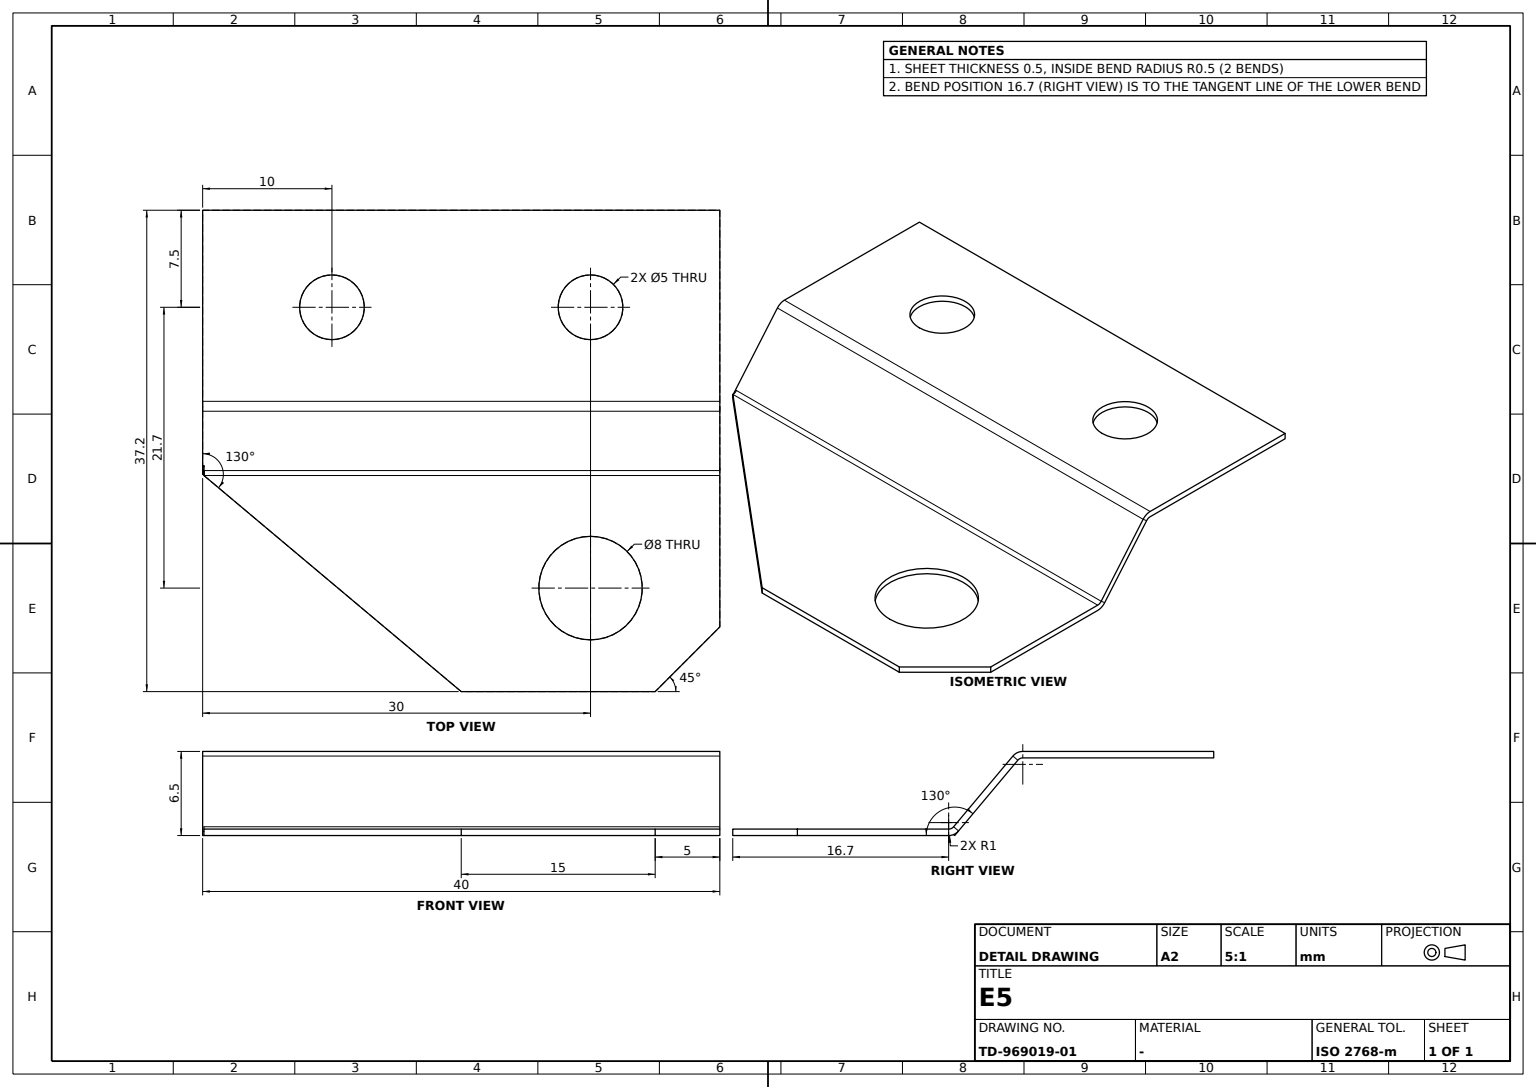
ISO-10303-21;
HEADER;
FILE_DESCRIPTION((''),'2;1');
FILE_NAME('','',(''),(''),'','','');
FILE_SCHEMA(('AUTOMOTIVE_DESIGN'));
ENDSEC;
DATA;
#1=APPLICATION_CONTEXT('');
#2=PRODUCT_CONTEXT('',#1,'mechanical');
#3=PRODUCT('','','',(#2));
#4=PRODUCT_DEFINITION_FORMATION('','',#3);
#5=PRODUCT_DEFINITION_CONTEXT('',#1,'design');
#6=PRODUCT_DEFINITION('','',#4,#5);
#7=PRODUCT_DEFINITION_SHAPE('','',#6);
#8=(LENGTH_UNIT()NAMED_UNIT(*)SI_UNIT(.MILLI.,.METRE.));
#9=(NAMED_UNIT(*)PLANE_ANGLE_UNIT()SI_UNIT($,.RADIAN.));
#10=(NAMED_UNIT(*)SI_UNIT($,.STERADIAN.)SOLID_ANGLE_UNIT());
#11=UNCERTAINTY_MEASURE_WITH_UNIT(LENGTH_MEASURE(0.005),#8,'distance_accuracy_value','');
#12=(GEOMETRIC_REPRESENTATION_CONTEXT(3)GLOBAL_UNCERTAINTY_ASSIGNED_CONTEXT((#11))GLOBAL_UNIT_ASSIGNED_CONTEXT((#8,#9,#10))REPRESENTATION_CONTEXT('',''));
#13=CARTESIAN_POINT('',(12.617883,-19.900744,-5.321394));
#14=VERTEX_POINT('',#13);
#15=CARTESIAN_POINT('',(12.617883,20.,-5.321394));
#16=VERTEX_POINT('',#15);
#17=CARTESIAN_POINT('',(12.617883,0.,-5.321394));
#18=DIRECTION('',(0.,1.,0.));
#19=VECTOR('',#18,1000.);
#20=LINE('',#17,#19);
#21=EDGE_CURVE('',#14,#16,#20,.T.);
#22=ORIENTED_EDGE('',*,*,#21,.F.);
#23=CARTESIAN_POINT('',(13.000905,-19.900744,-5.5));
#24=VERTEX_POINT('',#23);
#25=CARTESIAN_POINT('',(13.000905,-19.900744,-5.));
#26=DIRECTION('',(0.,0.,1.));
#27=AXIS2_PLACEMENT_3D('',#25,#18,#26);
#28=CIRCLE('',#27,0.5);
#29=EDGE_CURVE('',#14,#24,#28,.F.);
#30=ORIENTED_EDGE('',*,*,#29,.T.);
#31=CARTESIAN_POINT('',(13.000905,20.,-5.5));
#32=VERTEX_POINT('',#31);
#33=CARTESIAN_POINT('',(13.000905,0.,-5.5));
#34=LINE('',#33,#19);
#35=EDGE_CURVE('',#24,#32,#34,.T.);
#36=ORIENTED_EDGE('',*,*,#35,.T.);
#37=CARTESIAN_POINT('',(13.000905,20.,-5.));
#38=AXIS2_PLACEMENT_3D('',#37,#18,#26);
#39=CIRCLE('',#38,0.5);
#40=EDGE_CURVE('',#16,#32,#39,.F.);
#41=ORIENTED_EDGE('',*,*,#40,.F.);
#42=EDGE_LOOP('',(#22,#30,#36,#41));
#43=FACE_BOUND('',#42,.T.);
#44=CARTESIAN_POINT('',(13.000905,0.,-5.));
#45=DIRECTION('',(-0.766044443,0.,-0.64278761));
#46=AXIS2_PLACEMENT_3D('',#44,#18,#45);
#47=CYLINDRICAL_SURFACE('',#46,0.5);
#48=ADVANCED_FACE('',(#43),#47,.F.);
#49=ORIENTED_EDGE('',*,*,#21,.T.);
#50=CARTESIAN_POINT('',(8.032891,20.,0.142788));
#51=VERTEX_POINT('',#50);
#52=CARTESIAN_POINT('',(10.400321,20.,-2.678606));
#53=DIRECTION('',(0.64278761,0.,-0.766044443));
#54=VECTOR('',#53,1000.);
#55=LINE('',#52,#54);
#56=EDGE_CURVE('',#51,#16,#55,.T.);
#57=ORIENTED_EDGE('',*,*,#56,.F.);
#58=CARTESIAN_POINT('',(8.032891,-20.,0.142788));
#59=VERTEX_POINT('',#58);
#60=CARTESIAN_POINT('',(8.032891,0.,0.142788));
#61=DIRECTION('',(0.,-1.,0.));
#62=VECTOR('',#61,1000.);
#63=LINE('',#60,#62);
#64=EDGE_CURVE('',#51,#59,#63,.T.);
#65=ORIENTED_EDGE('',*,*,#64,.T.);
#66=CARTESIAN_POINT('',(12.91762,-20.,-5.678606));
#67=VERTEX_POINT('',#66);
#68=CARTESIAN_POINT('',(1.685384,-20.,7.707452));
#69=LINE('',#68,#54);
#70=EDGE_CURVE('',#59,#67,#69,.T.);
#71=ORIENTED_EDGE('',*,*,#70,.T.);
#72=CARTESIAN_POINT('',(12.91762,-19.900744,-5.678606));
#73=VERTEX_POINT('',#72);
#74=CARTESIAN_POINT('',(12.91762,0.,-5.678606));
#75=LINE('',#74,#62);
#76=EDGE_CURVE('',#73,#67,#75,.T.);
#77=ORIENTED_EDGE('',*,*,#76,.F.);
#78=CARTESIAN_POINT('',(7.883022,-19.900744,0.321394));
#79=DIRECTION('',(-0.64278761,0.,0.766044443));
#80=VECTOR('',#79,1000.);
#81=LINE('',#78,#80);
#82=EDGE_CURVE('',#73,#14,#81,.T.);
#83=ORIENTED_EDGE('',*,*,#82,.T.);
#84=EDGE_LOOP('',(#49,#57,#65,#71,#77,#83));
#85=FACE_BOUND('',#84,.T.);
#86=CARTESIAN_POINT('',(7.883022,0.,0.321394));
#87=AXIS2_PLACEMENT_3D('',#86,#45,#53);
#88=PLANE('',#87);
#89=ADVANCED_FACE('',(#85),#88,.F.);
#90=CARTESIAN_POINT('',(29.699613,15.,-6.));
#91=VERTEX_POINT('',#90);
#92=CARTESIAN_POINT('',(29.699613,15.,-5.5));
#93=VERTEX_POINT('',#92);
#94=VECTOR('',#26,1000.);
#95=LINE('',#90,#94);
#96=EDGE_CURVE('',#91,#93,#95,.T.);
#97=ORIENTED_EDGE('',*,*,#96,.T.);
#98=CARTESIAN_POINT('',(29.699613,0.,-5.5));
#99=VERTEX_POINT('',#98);
#100=LINE('',#98,#19);
#101=EDGE_CURVE('',#99,#93,#100,.T.);
#102=ORIENTED_EDGE('',*,*,#101,.F.);
#103=CARTESIAN_POINT('',(29.699613,0.,-6.));
#104=VERTEX_POINT('',#103);
#105=DIRECTION('',(0.,0.,-1.));
#106=VECTOR('',#105,1000.);
#107=LINE('',#103,#106);
#108=EDGE_CURVE('',#99,#104,#107,.T.);
#109=ORIENTED_EDGE('',*,*,#108,.T.);
#110=LINE('',#103,#19);
#111=EDGE_CURVE('',#104,#91,#110,.T.);
#112=ORIENTED_EDGE('',*,*,#111,.T.);
#113=EDGE_LOOP('',(#97,#102,#109,#112));
#114=FACE_BOUND('',#113,.T.);
#115=DIRECTION('',(1.,0.,0.));
#116=AXIS2_PLACEMENT_3D('',#103,#115,#18);
#117=PLANE('',#116);
#118=ADVANCED_FACE('',(#114),#117,.T.);
#119=CARTESIAN_POINT('',(7.266846,20.,0.));
#120=VERTEX_POINT('',#119);
#121=CARTESIAN_POINT('',(7.266846,-20.,0.));
#122=VERTEX_POINT('',#121);
#123=CARTESIAN_POINT('',(7.266846,0.,0.));
#124=LINE('',#123,#62);
#125=EDGE_CURVE('',#120,#122,#124,.T.);
#126=ORIENTED_EDGE('',*,*,#125,.F.);
#127=CARTESIAN_POINT('',(7.649868,20.,-0.178606));
#128=VERTEX_POINT('',#127);
#129=CARTESIAN_POINT('',(7.266846,20.,-0.5));
#130=AXIS2_PLACEMENT_3D('',#129,#61,#105);
#131=CIRCLE('',#130,0.5);
#132=EDGE_CURVE('',#128,#120,#131,.T.);
#133=ORIENTED_EDGE('',*,*,#132,.F.);
#134=CARTESIAN_POINT('',(7.649868,-20.,-0.178606));
#135=VERTEX_POINT('',#134);
#136=CARTESIAN_POINT('',(7.649868,0.,-0.178606));
#137=LINE('',#136,#62);
#138=EDGE_CURVE('',#128,#135,#137,.T.);
#139=ORIENTED_EDGE('',*,*,#138,.T.);
#140=CARTESIAN_POINT('',(7.266846,-20.,-0.5));
#141=AXIS2_PLACEMENT_3D('',#140,#61,#105);
#142=CIRCLE('',#141,0.5);
#143=EDGE_CURVE('',#122,#135,#142,.F.);
#144=ORIENTED_EDGE('',*,*,#143,.F.);
#145=EDGE_LOOP('',(#126,#133,#139,#144));
#146=FACE_BOUND('',#145,.T.);
#147=CARTESIAN_POINT('',(7.266846,0.,-0.5));
#148=AXIS2_PLACEMENT_3D('',#147,#61,#26);
#149=CYLINDRICAL_SURFACE('',#148,0.5);
#150=ADVANCED_FACE('',(#146),#149,.F.);
#151=ORIENTED_EDGE('',*,*,#125,.T.);
#152=CARTESIAN_POINT('',(-7.5,-20.,0.));
#153=VERTEX_POINT('',#152);
#154=CARTESIAN_POINT('',(0.,-20.,0.));
#155=VECTOR('',#115,1000.);
#156=LINE('',#154,#155);
#157=EDGE_CURVE('',#153,#122,#156,.T.);
#158=ORIENTED_EDGE('',*,*,#157,.F.);
#159=CARTESIAN_POINT('',(-7.5,20.,0.));
#160=VERTEX_POINT('',#159);
#161=LINE('',#159,#19);
#162=EDGE_CURVE('',#153,#160,#161,.T.);
#163=ORIENTED_EDGE('',*,*,#162,.T.);
#164=CARTESIAN_POINT('',(0.,20.,0.));
#165=LINE('',#164,#155);
#166=EDGE_CURVE('',#120,#160,#165,.F.);
#167=ORIENTED_EDGE('',*,*,#166,.F.);
#168=EDGE_LOOP('',(#151,#158,#163,#167));
#169=FACE_BOUND('',#168,.T.);
#170=CARTESIAN_POINT('',(2.5,-10.,0.));
#171=VERTEX_POINT('',#170);
#172=CARTESIAN_POINT('',(0.,-10.,0.));
#173=AXIS2_PLACEMENT_3D('',#172,#26,#115);
#174=CIRCLE('',#173,2.5);
#175=EDGE_CURVE('',#171,#171,#174,.T.);
#176=ORIENTED_EDGE('',*,*,#175,.T.);
#177=EDGE_LOOP('',(#176));
#178=FACE_BOUND('',#177,.T.);
#179=CARTESIAN_POINT('',(2.5,10.,0.));
#180=VERTEX_POINT('',#179);
#181=CARTESIAN_POINT('',(0.,10.,0.));
#182=AXIS2_PLACEMENT_3D('',#181,#26,#115);
#183=CIRCLE('',#182,2.5);
#184=EDGE_CURVE('',#180,#180,#183,.T.);
#185=ORIENTED_EDGE('',*,*,#184,.T.);
#186=EDGE_LOOP('',(#185));
#187=FACE_BOUND('',#186,.T.);
#188=CARTESIAN_POINT('',(0.,0.,0.));
#189=AXIS2_PLACEMENT_3D('',#188,#26,#18);
#190=PLANE('',#189);
#191=ADVANCED_FACE('',(#169,#178,#187),#190,.F.);
#192=ORIENTED_EDGE('',*,*,#157,.T.);
#193=CARTESIAN_POINT('',(7.266846,-20.,0.5));
#194=VERTEX_POINT('',#193);
#195=LINE('',#121,#94);
#196=EDGE_CURVE('',#122,#194,#195,.T.);
#197=ORIENTED_EDGE('',*,*,#196,.T.);
#198=CARTESIAN_POINT('',(-7.5,-20.,0.5));
#199=VERTEX_POINT('',#198);
#200=CARTESIAN_POINT('',(0.,-20.,0.5));
#201=LINE('',#200,#155);
#202=EDGE_CURVE('',#199,#194,#201,.T.);
#203=ORIENTED_EDGE('',*,*,#202,.F.);
#204=LINE('',#152,#106);
#205=EDGE_CURVE('',#199,#153,#204,.T.);
#206=ORIENTED_EDGE('',*,*,#205,.T.);
#207=EDGE_LOOP('',(#192,#197,#203,#206));
#208=FACE_BOUND('',#207,.T.);
#209=AXIS2_PLACEMENT_3D('',#152,#61,#115);
#210=PLANE('',#209);
#211=ADVANCED_FACE('',(#208),#210,.T.);
#212=CARTESIAN_POINT('',(24.699613,20.,-5.5));
#213=VERTEX_POINT('',#212);
#214=CARTESIAN_POINT('',(27.199613,17.5,-5.5));
#215=DIRECTION('',(-0.707106781,0.707106781,0.));
#216=VECTOR('',#215,1000.);
#217=LINE('',#214,#216);
#218=EDGE_CURVE('',#93,#213,#217,.T.);
#219=ORIENTED_EDGE('',*,*,#218,.F.);
#220=ORIENTED_EDGE('',*,*,#96,.F.);
#221=CARTESIAN_POINT('',(24.699613,20.,-6.));
#222=VERTEX_POINT('',#221);
#223=CARTESIAN_POINT('',(27.199613,17.5,-6.));
#224=LINE('',#223,#216);
#225=EDGE_CURVE('',#91,#222,#224,.T.);
#226=ORIENTED_EDGE('',*,*,#225,.T.);
#227=CARTESIAN_POINT('',(24.699613,20.,-2.839303));
#228=LINE('',#227,#106);
#229=EDGE_CURVE('',#222,#213,#228,.F.);
#230=ORIENTED_EDGE('',*,*,#229,.T.);
#231=EDGE_LOOP('',(#219,#220,#226,#230));
#232=FACE_BOUND('',#231,.T.);
#233=DIRECTION('',(-0.707106781,-0.707106781,0.));
#234=DIRECTION('',(0.707106781,-0.707106781,0.));
#235=AXIS2_PLACEMENT_3D('',#223,#233,#234);
#236=PLANE('',#235);
#237=ADVANCED_FACE('',(#232),#236,.F.);
#238=ORIENTED_EDGE('',*,*,#184,.F.);
#239=EDGE_LOOP('',(#238));
#240=FACE_BOUND('',#239,.T.);
#241=CARTESIAN_POINT('',(2.5,10.,0.5));
#242=VERTEX_POINT('',#241);
#243=CARTESIAN_POINT('',(0.,10.,0.5));
#244=AXIS2_PLACEMENT_3D('',#243,#26,#115);
#245=CIRCLE('',#244,2.5);
#246=EDGE_CURVE('',#242,#242,#245,.T.);
#247=ORIENTED_EDGE('',*,*,#246,.T.);
#248=EDGE_LOOP('',(#247));
#249=FACE_BOUND('',#248,.T.);
#250=CARTESIAN_POINT('',(0.,10.,0.25));
#251=AXIS2_PLACEMENT_3D('',#250,#105,#115);
#252=CYLINDRICAL_SURFACE('',#251,2.5);
#253=ADVANCED_FACE('',(#240,#249),#252,.F.);
#254=CARTESIAN_POINT('',(-7.5,20.,0.5));
#255=VERTEX_POINT('',#254);
#256=LINE('',#159,#94);
#257=EDGE_CURVE('',#255,#160,#256,.F.);
#258=ORIENTED_EDGE('',*,*,#257,.F.);
#259=CARTESIAN_POINT('',(7.266846,20.,0.5));
#260=VERTEX_POINT('',#259);
#261=CARTESIAN_POINT('',(0.,20.,0.5));
#262=LINE('',#261,#155);
#263=EDGE_CURVE('',#260,#255,#262,.F.);
#264=ORIENTED_EDGE('',*,*,#263,.F.);
#265=CARTESIAN_POINT('',(7.266846,20.,-2.839303));
#266=LINE('',#265,#94);
#267=EDGE_CURVE('',#120,#260,#266,.T.);
#268=ORIENTED_EDGE('',*,*,#267,.F.);
#269=ORIENTED_EDGE('',*,*,#166,.T.);
#270=EDGE_LOOP('',(#258,#264,#268,#269));
#271=FACE_BOUND('',#270,.T.);
#272=CARTESIAN_POINT('',(10.20881,20.,-2.839303));
#273=AXIS2_PLACEMENT_3D('',#272,#61,#115);
#274=PLANE('',#273);
#275=ADVANCED_FACE('',(#271),#274,.F.);
#276=CARTESIAN_POINT('',(2.5,-10.,0.5));
#277=VERTEX_POINT('',#276);
#278=CARTESIAN_POINT('',(0.,-10.,0.5));
#279=AXIS2_PLACEMENT_3D('',#278,#26,#115);
#280=CIRCLE('',#279,2.5);
#281=EDGE_CURVE('',#277,#277,#280,.T.);
#282=ORIENTED_EDGE('',*,*,#281,.F.);
#283=EDGE_LOOP('',(#282));
#284=FACE_BOUND('',#283,.T.);
#285=ORIENTED_EDGE('',*,*,#263,.T.);
#286=LINE('',#254,#19);
#287=EDGE_CURVE('',#199,#255,#286,.T.);
#288=ORIENTED_EDGE('',*,*,#287,.F.);
#289=ORIENTED_EDGE('',*,*,#202,.T.);
#290=CARTESIAN_POINT('',(7.266846,0.,0.5));
#291=LINE('',#290,#62);
#292=EDGE_CURVE('',#260,#194,#291,.T.);
#293=ORIENTED_EDGE('',*,*,#292,.F.);
#294=EDGE_LOOP('',(#285,#288,#289,#293));
#295=FACE_BOUND('',#294,.T.);
#296=ORIENTED_EDGE('',*,*,#246,.F.);
#297=EDGE_LOOP('',(#296));
#298=FACE_BOUND('',#297,.T.);
#299=CARTESIAN_POINT('',(0.,0.,0.5));
#300=AXIS2_PLACEMENT_3D('',#299,#26,#18);
#301=PLANE('',#300);
#302=ADVANCED_FACE('',(#284,#295,#298),#301,.T.);
#303=CARTESIAN_POINT('',(12.234861,-19.900744,-5.642788));
#304=VERTEX_POINT('',#303);
#305=CARTESIAN_POINT('',(13.000905,-19.900744,-6.));
#306=VERTEX_POINT('',#305);
#307=CIRCLE('',#27,1.);
#308=EDGE_CURVE('',#304,#306,#307,.F.);
#309=ORIENTED_EDGE('',*,*,#308,.T.);
#310=LINE('',#305,#94);
#311=EDGE_CURVE('',#306,#24,#310,.T.);
#312=ORIENTED_EDGE('',*,*,#311,.T.);
#313=ORIENTED_EDGE('',*,*,#29,.F.);
#314=DIRECTION('',(0.766044443,0.,0.64278761));
#315=VECTOR('',#314,1000.);
#316=LINE('',#303,#315);
#317=EDGE_CURVE('',#304,#14,#316,.T.);
#318=ORIENTED_EDGE('',*,*,#317,.F.);
#319=EDGE_LOOP('',(#309,#312,#313,#318));
#320=FACE_BOUND('',#319,.T.);
#321=CARTESIAN_POINT('',(12.965999,-19.900744,-5.5));
#322=CARTESIAN_POINT('',(12.931092,-19.900744,-6.));
#323=CARTESIAN_POINT('',(12.931092,-19.900744,-5.496954));
#324=CARTESIAN_POINT('',(12.861279,-19.900744,-5.993908));
#325=CARTESIAN_POINT('',(12.89654,-19.900744,-5.490861));
#326=CARTESIAN_POINT('',(12.792175,-19.900744,-5.981723));
#327=CARTESIAN_POINT('',(12.828854,-19.900744,-5.472709));
#328=CARTESIAN_POINT('',(12.656802,-19.900744,-5.945418));
#329=CARTESIAN_POINT('',(12.765334,-19.900744,-5.443106));
#330=CARTESIAN_POINT('',(12.529763,-19.900744,-5.886213));
#331=CARTESIAN_POINT('',(12.73495,-19.900744,-5.425564));
#332=CARTESIAN_POINT('',(12.468994,-19.900744,-5.851128));
#333=CARTESIAN_POINT('',(12.691903,-19.900744,-5.395408));
#334=CARTESIAN_POINT('',(12.3829,-19.900744,-5.790815));
#335=CARTESIAN_POINT('',(12.653261,-19.900744,-5.360001));
#336=CARTESIAN_POINT('',(12.305617,-19.900744,-5.720003));
#337=CARTESIAN_POINT('',(12.640904,-19.900744,-5.347644));
#338=CARTESIAN_POINT('',(12.280903,-19.900744,-5.695289));
#339=CARTESIAN_POINT('',(12.629102,-19.900744,-5.334764));
#340=CARTESIAN_POINT('',(12.257299,-19.900744,-5.669528));
#341=B_SPLINE_SURFACE_WITH_KNOTS('',5,1,((#23,#305),(#321,#322),(#323,#324),(#325,#326),(#327,#328),(#329,#330),(#331,#332),(#333,#334),(#335,#336),(#337,#338),(#339,#340),(#13,#303)),.RULED_SURF.,.F.,.F.,.F.,(6,3,3,6),(2,2),(0.,0.00112,0.00224,0.0028),(0.,0.00049),.UNSPECIFIED.);
#342=ADVANCED_FACE('',(#320),#341,.T.);
#343=ORIENTED_EDGE('',*,*,#132,.T.);
#344=ORIENTED_EDGE('',*,*,#267,.T.);
#345=CIRCLE('',#130,1.);
#346=EDGE_CURVE('',#51,#260,#345,.T.);
#347=ORIENTED_EDGE('',*,*,#346,.F.);
#348=LINE('',#127,#315);
#349=EDGE_CURVE('',#128,#51,#348,.T.);
#350=ORIENTED_EDGE('',*,*,#349,.F.);
#351=EDGE_LOOP('',(#343,#344,#347,#350));
#352=FACE_BOUND('',#351,.T.);
#353=CARTESIAN_POINT('',(7.301753,20.,0.));
#354=CARTESIAN_POINT('',(7.336659,20.,0.5));
#355=CARTESIAN_POINT('',(7.336659,20.,-0.003046));
#356=CARTESIAN_POINT('',(7.406473,20.,0.493908));
#357=CARTESIAN_POINT('',(7.371211,20.,-0.009139));
#358=CARTESIAN_POINT('',(7.475577,20.,0.481723));
#359=CARTESIAN_POINT('',(7.438898,20.,-0.027291));
#360=CARTESIAN_POINT('',(7.61095,20.,0.445418));
#361=CARTESIAN_POINT('',(7.502417,20.,-0.056894));
#362=CARTESIAN_POINT('',(7.737988,20.,0.386213));
#363=CARTESIAN_POINT('',(7.532802,20.,-0.074436));
#364=CARTESIAN_POINT('',(7.798758,20.,0.351128));
#365=CARTESIAN_POINT('',(7.575849,20.,-0.104592));
#366=CARTESIAN_POINT('',(7.884852,20.,0.290815));
#367=CARTESIAN_POINT('',(7.61449,20.,-0.139999));
#368=CARTESIAN_POINT('',(7.962135,20.,0.220003));
#369=CARTESIAN_POINT('',(7.626847,20.,-0.152356));
#370=CARTESIAN_POINT('',(7.986849,20.,0.195289));
#371=CARTESIAN_POINT('',(7.63865,20.,-0.165236));
#372=CARTESIAN_POINT('',(8.010453,20.,0.169528));
#373=B_SPLINE_SURFACE_WITH_KNOTS('',5,1,((#119,#259),(#353,#354),(#355,#356),(#357,#358),(#359,#360),(#361,#362),(#363,#364),(#365,#366),(#367,#368),(#369,#370),(#371,#372),(#127,#50)),.RULED_SURF.,.F.,.F.,.F.,(6,3,3,6),(2,2),(0.,0.00112,0.00224,0.0028),(0.,0.00049),.UNSPECIFIED.);
#374=ADVANCED_FACE('',(#352),#373,.F.);
#375=CARTESIAN_POINT('',(12.234861,20.,-5.642788));
#376=VERTEX_POINT('',#375);
#377=VECTOR('',#45,1000.);
#378=LINE('',#15,#377);
#379=EDGE_CURVE('',#376,#16,#378,.F.);
#380=ORIENTED_EDGE('',*,*,#379,.F.);
#381=CARTESIAN_POINT('',(10.017299,20.,-3.));
#382=LINE('',#381,#54);
#383=EDGE_CURVE('',#128,#376,#382,.T.);
#384=ORIENTED_EDGE('',*,*,#383,.F.);
#385=ORIENTED_EDGE('',*,*,#349,.T.);
#386=ORIENTED_EDGE('',*,*,#56,.T.);
#387=EDGE_LOOP('',(#380,#384,#385,#386));
#388=FACE_BOUND('',#387,.T.);
#389=ADVANCED_FACE('',(#388),#274,.F.);
#390=CARTESIAN_POINT('',(25.699613,10.,-6.));
#391=VERTEX_POINT('',#390);
#392=CARTESIAN_POINT('',(21.699613,10.,-6.));
#393=AXIS2_PLACEMENT_3D('',#392,#26,#115);
#394=CIRCLE('',#393,4.);
#395=EDGE_CURVE('',#391,#391,#394,.T.);
#396=ORIENTED_EDGE('',*,*,#395,.F.);
#397=EDGE_LOOP('',(#396));
#398=FACE_BOUND('',#397,.T.);
#399=CARTESIAN_POINT('',(25.699613,10.,-5.5));
#400=VERTEX_POINT('',#399);
#401=CARTESIAN_POINT('',(21.699613,10.,-5.5));
#402=AXIS2_PLACEMENT_3D('',#401,#26,#115);
#403=CIRCLE('',#402,4.);
#404=EDGE_CURVE('',#400,#400,#403,.T.);
#405=ORIENTED_EDGE('',*,*,#404,.T.);
#406=EDGE_LOOP('',(#405));
#407=FACE_BOUND('',#406,.T.);
#408=CARTESIAN_POINT('',(21.699613,10.,-5.75));
#409=AXIS2_PLACEMENT_3D('',#408,#105,#115);
#410=CYLINDRICAL_SURFACE('',#409,4.);
#411=ADVANCED_FACE('',(#398,#407),#410,.F.);
#412=CARTESIAN_POINT('',(13.000905,20.,-6.));
#413=VERTEX_POINT('',#412);
#414=CARTESIAN_POINT('',(13.000905,20.,-2.839303));
#415=LINE('',#414,#94);
#416=EDGE_CURVE('',#413,#32,#415,.T.);
#417=ORIENTED_EDGE('',*,*,#416,.T.);
#418=CARTESIAN_POINT('',(0.,20.,-5.5));
#419=LINE('',#418,#155);
#420=EDGE_CURVE('',#213,#32,#419,.F.);
#421=ORIENTED_EDGE('',*,*,#420,.F.);
#422=ORIENTED_EDGE('',*,*,#229,.F.);
#423=CARTESIAN_POINT('',(0.,20.,-6.));
#424=LINE('',#423,#155);
#425=EDGE_CURVE('',#222,#413,#424,.F.);
#426=ORIENTED_EDGE('',*,*,#425,.T.);
#427=EDGE_LOOP('',(#417,#421,#422,#426));
#428=FACE_BOUND('',#427,.T.);
#429=ADVANCED_FACE('',(#428),#274,.F.);
#430=ORIENTED_EDGE('',*,*,#143,.T.);
#431=LINE('',#58,#377);
#432=EDGE_CURVE('',#135,#59,#431,.F.);
#433=ORIENTED_EDGE('',*,*,#432,.T.);
#434=CIRCLE('',#141,1.);
#435=EDGE_CURVE('',#194,#59,#434,.F.);
#436=ORIENTED_EDGE('',*,*,#435,.F.);
#437=ORIENTED_EDGE('',*,*,#196,.F.);
#438=EDGE_LOOP('',(#430,#433,#436,#437));
#439=FACE_BOUND('',#438,.T.);
#440=CARTESIAN_POINT('',(7.301753,-20.,0.));
#441=CARTESIAN_POINT('',(7.336659,-20.,0.5));
#442=CARTESIAN_POINT('',(7.336659,-20.,-0.003046));
#443=CARTESIAN_POINT('',(7.406473,-20.,0.493908));
#444=CARTESIAN_POINT('',(7.371211,-20.,-0.009139));
#445=CARTESIAN_POINT('',(7.475577,-20.,0.481723));
#446=CARTESIAN_POINT('',(7.438898,-20.,-0.027291));
#447=CARTESIAN_POINT('',(7.61095,-20.,0.445418));
#448=CARTESIAN_POINT('',(7.502417,-20.,-0.056894));
#449=CARTESIAN_POINT('',(7.737988,-20.,0.386213));
#450=CARTESIAN_POINT('',(7.532802,-20.,-0.074436));
#451=CARTESIAN_POINT('',(7.798758,-20.,0.351128));
#452=CARTESIAN_POINT('',(7.575849,-20.,-0.104592));
#453=CARTESIAN_POINT('',(7.884852,-20.,0.290815));
#454=CARTESIAN_POINT('',(7.61449,-20.,-0.139999));
#455=CARTESIAN_POINT('',(7.962135,-20.,0.220003));
#456=CARTESIAN_POINT('',(7.626847,-20.,-0.152356));
#457=CARTESIAN_POINT('',(7.986849,-20.,0.195289));
#458=CARTESIAN_POINT('',(7.63865,-20.,-0.165236));
#459=CARTESIAN_POINT('',(8.010453,-20.,0.169528));
#460=B_SPLINE_SURFACE_WITH_KNOTS('',5,1,((#121,#193),(#440,#441),(#442,#443),(#444,#445),(#446,#447),(#448,#449),(#450,#451),(#452,#453),(#454,#455),(#456,#457),(#458,#459),(#134,#58)),.RULED_SURF.,.F.,.F.,.F.,(6,3,3,6),(2,2),(0.,0.00112,0.00224,0.0028),(0.,0.00049),.UNSPECIFIED.);
#461=ADVANCED_FACE('',(#439),#460,.T.);
#462=ORIENTED_EDGE('',*,*,#287,.T.);
#463=ORIENTED_EDGE('',*,*,#257,.T.);
#464=ORIENTED_EDGE('',*,*,#162,.F.);
#465=ORIENTED_EDGE('',*,*,#205,.F.);
#466=EDGE_LOOP('',(#462,#463,#464,#465));
#467=FACE_BOUND('',#466,.T.);
#468=DIRECTION('',(-1.,0.,0.));
#469=AXIS2_PLACEMENT_3D('',#159,#468,#61);
#470=PLANE('',#469);
#471=ADVANCED_FACE('',(#467),#470,.T.);
#472=ORIENTED_EDGE('',*,*,#416,.F.);
#473=CIRCLE('',#38,1.);
#474=EDGE_CURVE('',#376,#413,#473,.F.);
#475=ORIENTED_EDGE('',*,*,#474,.F.);
#476=ORIENTED_EDGE('',*,*,#379,.T.);
#477=ORIENTED_EDGE('',*,*,#40,.T.);
#478=EDGE_LOOP('',(#472,#475,#476,#477));
#479=FACE_BOUND('',#478,.T.);
#480=CARTESIAN_POINT('',(12.640321,20.,-5.348134));
#481=CARTESIAN_POINT('',(12.279736,20.,-5.696268));
#482=CARTESIAN_POINT('',(12.665092,20.,-5.372916));
#483=CARTESIAN_POINT('',(12.329278,20.,-5.745832));
#484=CARTESIAN_POINT('',(12.691969,20.,-5.395468));
#485=CARTESIAN_POINT('',(12.383032,20.,-5.790936));
#486=CARTESIAN_POINT('',(12.749382,20.,-5.435651));
#487=CARTESIAN_POINT('',(12.497859,20.,-5.871302));
#488=CARTESIAN_POINT('',(12.812889,20.,-5.465281));
#489=CARTESIAN_POINT('',(12.624872,20.,-5.930562));
#490=CARTESIAN_POINT('',(12.845858,20.,-5.477281));
#491=CARTESIAN_POINT('',(12.69081,20.,-5.954562));
#492=CARTESIAN_POINT('',(12.896629,20.,-5.490873));
#493=CARTESIAN_POINT('',(12.792352,20.,-5.981746));
#494=CARTESIAN_POINT('',(12.94859,20.,-5.497715));
#495=CARTESIAN_POINT('',(12.896274,20.,-5.995431));
#496=CARTESIAN_POINT('',(12.965999,20.,-5.499238));
#497=CARTESIAN_POINT('',(12.931092,20.,-5.998477));
#498=CARTESIAN_POINT('',(12.983452,20.,-5.5));
#499=CARTESIAN_POINT('',(12.965999,20.,-6.));
#500=B_SPLINE_SURFACE_WITH_KNOTS('',5,1,((#15,#375),(#480,#481),(#482,#483),(#484,#485),(#486,#487),(#488,#489),(#490,#491),(#492,#493),(#494,#495),(#496,#497),(#498,#499),(#31,#412)),.RULED_SURF.,.F.,.F.,.F.,(6,3,3,6),(2,2),(0.,0.00112,0.00224,0.0028),(0.,0.00049),.UNSPECIFIED.);
#501=ADVANCED_FACE('',(#479),#500,.T.);
#502=CARTESIAN_POINT('',(12.534598,-20.,-6.));
#503=VERTEX_POINT('',#502);
#504=CARTESIAN_POINT('',(1.302361,-20.,7.386058));
#505=LINE('',#504,#54);
#506=EDGE_CURVE('',#135,#503,#505,.T.);
#507=ORIENTED_EDGE('',*,*,#506,.T.);
#508=CARTESIAN_POINT('',(12.726109,-20.,-5.839303));
#509=LINE('',#508,#315);
#510=EDGE_CURVE('',#503,#67,#509,.T.);
#511=ORIENTED_EDGE('',*,*,#510,.T.);
#512=ORIENTED_EDGE('',*,*,#70,.F.);
#513=ORIENTED_EDGE('',*,*,#432,.F.);
#514=EDGE_LOOP('',(#507,#511,#512,#513));
#515=FACE_BOUND('',#514,.T.);
#516=ADVANCED_FACE('',(#515),#210,.T.);
#517=ORIENTED_EDGE('',*,*,#317,.T.);
#518=ORIENTED_EDGE('',*,*,#82,.F.);
#519=CARTESIAN_POINT('',(12.534598,-19.900744,-6.));
#520=VERTEX_POINT('',#519);
#521=CARTESIAN_POINT('',(12.726109,-19.900744,-5.839303));
#522=LINE('',#521,#315);
#523=EDGE_CURVE('',#520,#73,#522,.T.);
#524=ORIENTED_EDGE('',*,*,#523,.F.);
#525=CARTESIAN_POINT('',(7.5,-19.900744,0.));
#526=LINE('',#525,#80);
#527=EDGE_CURVE('',#520,#304,#526,.T.);
#528=ORIENTED_EDGE('',*,*,#527,.T.);
#529=EDGE_LOOP('',(#517,#518,#524,#528));
#530=FACE_BOUND('',#529,.T.);
#531=CARTESIAN_POINT('',(12.384729,-19.900744,-5.821394));
#532=AXIS2_PLACEMENT_3D('',#531,#61,#115);
#533=PLANE('',#532);
#534=ADVANCED_FACE('',(#530),#533,.F.);
#535=CARTESIAN_POINT('',(12.534598,0.,-6.));
#536=LINE('',#535,#62);
#537=EDGE_CURVE('',#520,#503,#536,.T.);
#538=ORIENTED_EDGE('',*,*,#537,.T.);
#539=ORIENTED_EDGE('',*,*,#506,.F.);
#540=ORIENTED_EDGE('',*,*,#138,.F.);
#541=ORIENTED_EDGE('',*,*,#383,.T.);
#542=CARTESIAN_POINT('',(12.234861,0.,-5.642788));
#543=LINE('',#542,#19);
#544=EDGE_CURVE('',#304,#376,#543,.T.);
#545=ORIENTED_EDGE('',*,*,#544,.F.);
#546=ORIENTED_EDGE('',*,*,#527,.F.);
#547=EDGE_LOOP('',(#538,#539,#540,#541,#545,#546));
#548=FACE_BOUND('',#547,.T.);
#549=CARTESIAN_POINT('',(7.5,0.,0.));
#550=AXIS2_PLACEMENT_3D('',#549,#45,#53);
#551=PLANE('',#550);
#552=ADVANCED_FACE('',(#548),#551,.T.);
#553=ORIENTED_EDGE('',*,*,#510,.F.);
#554=ORIENTED_EDGE('',*,*,#537,.F.);
#555=ORIENTED_EDGE('',*,*,#523,.T.);
#556=ORIENTED_EDGE('',*,*,#76,.T.);
#557=EDGE_LOOP('',(#553,#554,#555,#556));
#558=FACE_BOUND('',#557,.T.);
#559=CARTESIAN_POINT('',(12.726109,0.,-5.839303));
#560=AXIS2_PLACEMENT_3D('',#559,#79,#314);
#561=PLANE('',#560);
#562=ADVANCED_FACE('',(#558),#561,.F.);
#563=ORIENTED_EDGE('',*,*,#435,.T.);
#564=ORIENTED_EDGE('',*,*,#64,.F.);
#565=ORIENTED_EDGE('',*,*,#346,.T.);
#566=ORIENTED_EDGE('',*,*,#292,.T.);
#567=EDGE_LOOP('',(#563,#564,#565,#566));
#568=FACE_BOUND('',#567,.T.);
#569=CYLINDRICAL_SURFACE('',#148,1.);
#570=ADVANCED_FACE('',(#568),#569,.T.);
#571=ORIENTED_EDGE('',*,*,#281,.T.);
#572=EDGE_LOOP('',(#571));
#573=FACE_BOUND('',#572,.T.);
#574=ORIENTED_EDGE('',*,*,#175,.F.);
#575=EDGE_LOOP('',(#574));
#576=FACE_BOUND('',#575,.T.);
#577=CARTESIAN_POINT('',(0.,-10.,0.25));
#578=AXIS2_PLACEMENT_3D('',#577,#105,#115);
#579=CYLINDRICAL_SURFACE('',#578,2.5);
#580=ADVANCED_FACE('',(#573,#576),#579,.F.);
#581=ORIENTED_EDGE('',*,*,#35,.F.);
#582=CARTESIAN_POINT('',(17.428448,-14.624204,-5.5));
#583=DIRECTION('',(0.64278761,0.766044443,0.));
#584=VECTOR('',#583,1000.);
#585=LINE('',#582,#584);
#586=EDGE_CURVE('',#24,#99,#585,.T.);
#587=ORIENTED_EDGE('',*,*,#586,.T.);
#588=ORIENTED_EDGE('',*,*,#101,.T.);
#589=ORIENTED_EDGE('',*,*,#218,.T.);
#590=ORIENTED_EDGE('',*,*,#420,.T.);
#591=EDGE_LOOP('',(#581,#587,#588,#589,#590));
#592=FACE_BOUND('',#591,.T.);
#593=ORIENTED_EDGE('',*,*,#404,.F.);
#594=EDGE_LOOP('',(#593));
#595=FACE_BOUND('',#594,.T.);
#596=CARTESIAN_POINT('',(0.,0.,-5.5));
#597=AXIS2_PLACEMENT_3D('',#596,#26,#18);
#598=PLANE('',#597);
#599=ADVANCED_FACE('',(#592,#595),#598,.T.);
#600=ORIENTED_EDGE('',*,*,#586,.F.);
#601=ORIENTED_EDGE('',*,*,#311,.F.);
#602=CARTESIAN_POINT('',(17.428448,-14.624204,-6.));
#603=LINE('',#602,#584);
#604=EDGE_CURVE('',#306,#104,#603,.T.);
#605=ORIENTED_EDGE('',*,*,#604,.T.);
#606=ORIENTED_EDGE('',*,*,#108,.F.);
#607=EDGE_LOOP('',(#600,#601,#605,#606));
#608=FACE_BOUND('',#607,.T.);
#609=CARTESIAN_POINT('',(12.91762,-20.,-6.));
#610=DIRECTION('',(0.766044443,-0.64278761,0.));
#611=AXIS2_PLACEMENT_3D('',#609,#610,#583);
#612=PLANE('',#611);
#613=ADVANCED_FACE('',(#608),#612,.T.);
#614=ORIENTED_EDGE('',*,*,#395,.T.);
#615=EDGE_LOOP('',(#614));
#616=FACE_BOUND('',#615,.T.);
#617=CARTESIAN_POINT('',(13.000905,0.,-6.));
#618=LINE('',#617,#19);
#619=EDGE_CURVE('',#306,#413,#618,.T.);
#620=ORIENTED_EDGE('',*,*,#619,.T.);
#621=ORIENTED_EDGE('',*,*,#425,.F.);
#622=ORIENTED_EDGE('',*,*,#225,.F.);
#623=ORIENTED_EDGE('',*,*,#111,.F.);
#624=ORIENTED_EDGE('',*,*,#604,.F.);
#625=EDGE_LOOP('',(#620,#621,#622,#623,#624));
#626=FACE_BOUND('',#625,.T.);
#627=CARTESIAN_POINT('',(0.,0.,-6.));
#628=AXIS2_PLACEMENT_3D('',#627,#26,#18);
#629=PLANE('',#628);
#630=ADVANCED_FACE('',(#616,#626),#629,.F.);
#631=ORIENTED_EDGE('',*,*,#474,.T.);
#632=ORIENTED_EDGE('',*,*,#619,.F.);
#633=ORIENTED_EDGE('',*,*,#308,.F.);
#634=ORIENTED_EDGE('',*,*,#544,.T.);
#635=EDGE_LOOP('',(#631,#632,#633,#634));
#636=FACE_BOUND('',#635,.T.);
#637=CYLINDRICAL_SURFACE('',#46,1.);
#638=ADVANCED_FACE('',(#636),#637,.T.);
#639=CLOSED_SHELL('',(#48,#89,#118,#150,#191,#211,#237,#253,#275,#302,#342,#374,#389,#411,#429,#461,#471,#501,#516,#534,#552,#562,#570,#580,#599,#613,#630,#638));
#640=MANIFOLD_SOLID_BREP('',#639);
#641=ADVANCED_BREP_SHAPE_REPRESENTATION('',(#640),#12);
#642=SHAPE_DEFINITION_REPRESENTATION(#7,#641);
ENDSEC;
END-ISO-10303-21;
